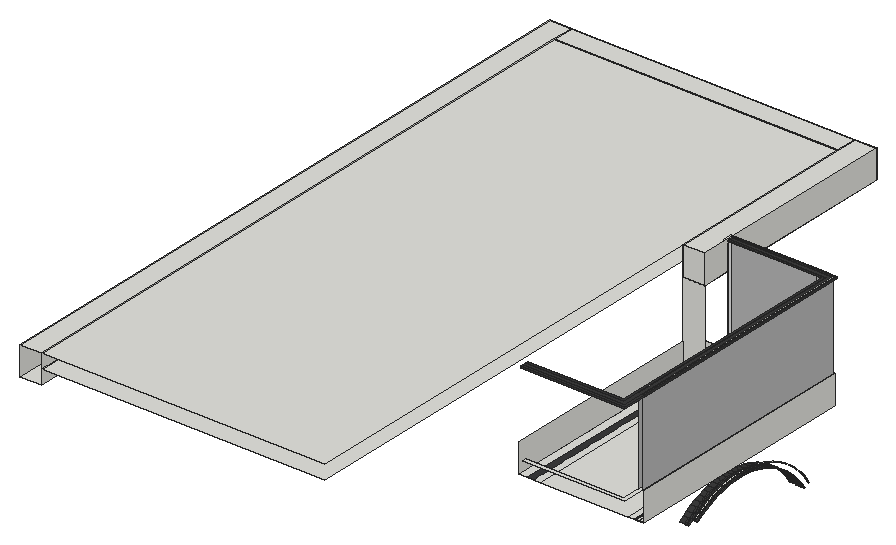
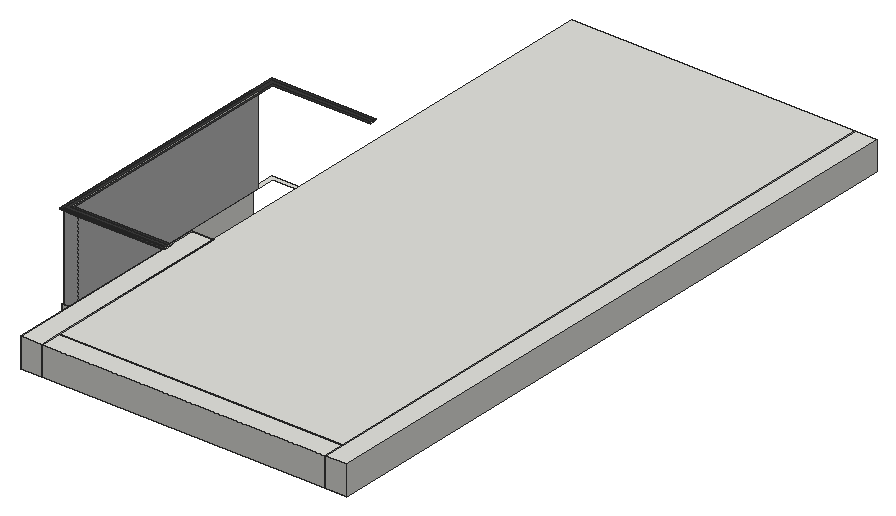
# SketchUp Ruby script. Lengths in inches.
U = 1.inch
M = Sketchup.active_model
def pt(a) = Geom::Point3d.new(a.map { |v| v * U })
def face(e, loops, mat)
  f = e.add_face(loops[0].map { |a| pt(a) })
  loops[1..].each { |l| e.add_face(l.map { |a| pt(a) }).erase! }
  f.material = f.back_material = mat if mat
  f
end
# faces: each face lists its corners as indices into pts; further lists are holes
def faces(e, pts, list, mat = nil) = list.each { |f| face(e, (f[0].is_a?(Array) ? f : [f]).map { |l| l.map { |i| pts[i] } }, mat) }
# xy, xz, yz: faces in a plane at the given z, y or x. An outline is a flat list of corners, or four numbers for a rectangle; further outlines are holes
def ring(l) = l.size == 4 ? [[l[0], l[1]], [l[2], l[1]], [l[2], l[3]], [l[0], l[3]]] : l.each_slice(2).to_a
def flat(e, list, mat, &to3) = list.each { |f| face(e, (f[0].is_a?(Array) ? f : [f]).map { |l| ring(l).map { |u, v| to3.(u, v) } }, mat) }
def xy(e, z, list, mat = nil) = flat(e, list, mat) { |x, y| [x, y, z] }
def xz(e, y, list, mat = nil) = flat(e, list, mat) { |x, z| [x, y, z] }
def yz(e, x, list, mat = nil) = flat(e, list, mat) { |y, z| [x, y, z] }
def lines(e, pts, list) = list.each { |a, b| e.add_line(pt(pts[a]), pt(pts[b])) }
# prism: a flat outline (further loops are holes) pulled along v
def prism(e, loops, v, mat = nil)
  f = face(e, loops, mat); d = Geom::Vector3d.new(v.map { |x| x * U })
  f.pushpull(f.normal.samedirection?(d) ? d.length : -d.length)
end
def box(e, o, s, mat = nil) = prism(e, [[o, [o[0] + s[0], o[1], o[2]], [o[0] + s[0], o[1] + s[1], o[2]], [o[0], o[1] + s[1], o[2]]]], [0, 0, s[2]], mat)
def at(x, y, z, deg = 0) = Geom::Transformation.translation(pt([x, y, z])) * Geom::Transformation.rotation(ORIGIN, Z_AXIS, deg.degrees)
def axes(o, x, y, z) = Geom::Transformation.new([*x, 0, *y, 0, *z, 0, *pt(o).to_a, 1])
def part(name) = M.definitions.add(name)
# library, detail: a bought-in or finely detailed component or shape, given as its bounding box
def library(name, o, s) = part(name).tap { |d| box(d.entities, o, s) }
def detail(e, o, s) = box(e.add_group.entities, o, s)
def put(e, d, t, mat = nil) = e.add_instance(d, t).tap { |i| i.material = mat if mat }
def group(e, t, mat = nil) = e.add_group.tap { |g| g.transformation = t; g.material = mat if mat }.entities
root = M.entities
M.materials.add("[Color M07]").color = [58, 58, 58]
M.materials.add("[Mirror 01]").color = [185, 185, 185]
M.materials.add("[Mirror 02]").color = [229, 229, 229]
xy(root,336.73,[[150.22,149.02,151.47,169.15],[150.22,172.14,151.47,188.97],[150.22,191.96,151.47,209.51]],"[Color M07]")
xy(root,337.6875,[[145.27,124.96,145.27,215.22,190.96,215.22,190.96,124.96,154.46,124.96,154.46,210.47,145.46,210.47,145.46,124.96],[145.46,124.96,148.9,210.47],[151.47,124.96,154.46,210.47],[190.96,124.96,193.21,224.6],[193.21,124.96,193.59,224.6],
  [193.59,124.96,193.96,224.6],[193.96,124.96,194.34,224.6],[194.34,124.96,194.71,224.6],[194.71,124.96,195.09,224.6],[195.09,124.96,195.46,224.6],
  [195.46,124.96,195.84,224.6],[195.84,124.96,196.21,224.6],[196.21,124.96,196.59,224.6],[196.59,124.96,197.34,224.6]])
xy(root,337.6875,[[148.9,124.96,151.47,210.47]],"[Color M07]")
xy(root,349.6875,[[154.46,115.71,154.46,117.49,195.18,117.49,195.18,222.44,154.46,222.44,154.46,224.22,196.96,224.22,196.96,115.71],[196.96,124.96,197.34,224.6],[154.46,224.22,190.96,224.6],[190.96,224.22,196.96,224.6]])
xy(root,373.6875,[[18.46,24,27.46,299.8125],[145.46,210.47,154.46,299.8125],[27.46,290.8125,145.46,299.8125]])
xy(root,379.6875,[[27.46,24,145.46,290.8125]])
xy(root,385.0625,[[154.46,115.71,154.46,117.49,195.18,117.49,195.18,222.44,154.46,222.44,154.46,224.22,196.96,224.22,196.96,115.71]])
xy(root,385.0625,[[154.46,114.76,154.46,115.71,196.96,115.71,196.96,224.22,154.46,224.22,154.46,225.17,197.91,225.17,197.91,114.76]],"[Color M07]")
xy(root,385.6875,[[18.46,24,27.46,299.8125],[27.46,24,145.46,290.8125],[145.46,210.47,154.46,210.47,154.46,221.49,153.51,221.49,153.51,225.17,154.46,225.17,154.46,299.8125,145.46,299.8125],[153.51,221.49,154.46,225.17],[27.46,290.8125,145.46,299.8125]])
xy(root,385.6875,[[154.46,114.76,197.91,114.76,197.91,225.17,154.46,225.17,154.46,224.22,196.96,224.22,196.96,115.71,154.46,115.71],[154.46,115.71,196.96,115.71,196.96,224.22,154.46,224.22,154.46,222.44,195.18,222.44,195.18,117.49,154.46,117.49],[154.46,117.49,195.18,117.49,195.18,222.44,154.46,222.44,154.46,221.49,194.23,221.49,194.23,118.4375,154.46,118.4375]],"[Color M07]")
xz(root,210.47,[[145.46,337.6875,154.46,373.6875],[145.46,373.6875,154.46,385.6875]])
xz(root,215.22,[[145.27,337.6875,154.46,349.6875]])
xz(root,222.44,[[190.96,385.0625,195.18,385.6875]])
xz(root,222.44,[[154.46,385.0625,156.24,385.6875],[156.24,385.0625,190.96,385.6875]],"[Color M07]")
xz(root,222.44,[[156.24,349.6875,190.96,385.0625],[190.96,349.6875,195.18,385.0625]],"[Mirror 01]")
xz(root,222.44,[[154.46,349.6875,156.24,385.0625]],"[Mirror 02]")
xz(root,224.22,[[154.46,385.0625,190.96,385.6875],[190.96,385.0625,196.96,385.6875]])
xz(root,224.22,[[154.46,349.6875,190.96,385.0625],[190.96,349.6875,196.96,385.0625]],"[Mirror 01]")
xz(root,224.6,[[190.96,337.6875,197.34,349.6875]])
xz(root,225.17,[[154.46,385.0625,190.96,385.6875],[190.96,385.0625,197.91,385.6875]],"[Color M07]")
xz(root,290.8125,[[27.46,373.6875,145.46,379.6875],[27.46,379.6875,145.46,385.6875]])
xz(root,299.8125,[[18.46,373.6875,27.46,385.6875],[27.46,373.6875,145.46,385.6875],[145.46,373.6875,154.46,385.6875]])
yz(root,18.46,[[24,373.6875,299.8125,385.6875]])
yz(root,27.46,[[24,373.6875,290.8125,379.6875],[290.8125,373.6875,299.8125,385.6875],[24,379.6875,290.8125,385.6875]])
yz(root,145.27,[[124.96,337.6875,215.22,349.6875]])
yz(root,145.46,[[210.47,373.6875,290.8125,379.6875],[290.8125,373.6875,299.8125,385.6875],[210.47,379.6875,290.8125,385.6875]])
yz(root,154.46,[[222.44,349.6875,224.22,373.6875],[210.47,373.6875,222.44,385.6875],[222.44,373.6875,224.22,385.0625],[224.22,373.6875,299.8125,373.6875,299.8125,385.6875,225.17,385.6875,225.17,385.0625,224.22,385.0625],[222.44,385.0625,224.22,385.6875],
  [224.22,385.0625,225.17,385.6875]])
yz(root,195.18,[[124.96,385.0625,222.44,385.6875]])
yz(root,195.18,[[124.96,349.6875,222.44,385.0625]],"[Mirror 01]")
yz(root,196.96,[[124.96,385.0625,224.22,385.6875]])
yz(root,196.96,[[124.96,349.6875,224.22,385.0625]],"[Mirror 01]")
yz(root,197.34,[[124.96,337.6875,224.6,349.6875]])
yz(root,197.91,[[124.96,385.0625,225.17,385.6875]],"[Color M07]")
p = [[190.96,209.22,313.61],[193.21,209.22,313.61],[193.21,207.91,315.55],[190.96,207.91,315.55],[193.59,207.91,315.55],[193.59,209.22,313.61],
  [193.96,207.91,315.55],[193.96,209.22,313.61],[194.34,207.91,315.55],[194.34,209.22,313.61],[194.71,207.91,315.55],[194.71,209.22,313.61],
  [195.09,207.91,315.55],[195.09,209.22,313.61],[195.46,207.91,315.55],[195.46,209.22,313.61],[195.84,207.91,315.55],[195.84,209.22,313.61],
  [196.21,207.91,315.55],[196.21,209.22,313.61],[196.59,207.91,315.55],[196.59,209.22,313.61],[196.96,207.91,315.55],[196.96,209.22,313.61],
  [196.96,209.77,316.88],[196.96,211.15,314.82],[197.34,211.15,314.82],[197.34,209.77,316.88],[193.21,206.49,317.42],[190.96,206.49,317.42],
  [193.59,206.49,317.42],[193.96,206.49,317.42],[194.34,206.49,317.42],[194.71,206.49,317.42],[195.09,206.49,317.42],[195.46,206.49,317.42],
  [195.84,206.49,317.42],[196.21,206.49,317.42],[196.59,206.49,317.42],[196.96,206.49,317.42],[196.96,208.26,318.85],[197.34,208.26,318.85],
  [193.21,204.96,319.19],[190.96,204.96,319.19],[193.59,204.96,319.19],[193.96,204.96,319.19],[194.34,204.96,319.19],[194.71,204.96,319.19],
  [195.09,204.96,319.19],[195.46,204.96,319.19],[195.84,204.96,319.19],[196.21,204.96,319.19],[196.59,204.96,319.19],[196.96,204.96,319.19],
  [196.96,206.65,320.73],[197.34,206.65,320.73],[193.21,203.33,320.88],[190.96,203.33,320.88],[193.59,203.33,320.88],[193.96,203.33,320.88],
  [194.34,203.33,320.88],[194.71,203.33,320.88],[195.09,203.33,320.88],[195.46,203.33,320.88],[195.84,203.33,320.88],[196.21,203.33,320.88],
  [196.59,203.33,320.88],[196.96,203.33,320.88],[196.96,204.92,322.51],[197.34,204.92,322.51],[193.21,201.6,322.46],[190.96,201.6,322.46],
  [193.59,201.6,322.46],[193.96,201.6,322.46],[194.34,201.6,322.46],[194.71,201.6,322.46],[195.09,201.6,322.46],[195.46,201.6,322.46],
  [195.84,201.6,322.46],[196.21,201.6,322.46],[196.59,201.6,322.46],[196.96,201.6,322.46],[193.21,199.79,323.9375],[190.96,199.79,323.9375],
  [193.59,199.79,323.9375],[193.96,199.79,323.9375],[194.34,199.79,323.9375],[194.71,199.79,323.9375],[195.09,199.79,323.9375],[195.46,199.79,323.9375],
  [195.84,199.79,323.9375],[196.21,199.79,323.9375],[196.59,199.79,323.9375],[196.96,199.79,323.9375],[196.96,203.1,324.1875],[197.34,203.1,324.1875],
  [190.96,153.71,325.31],[193.21,153.71,325.31],[193.21,151.81,323.9375],[190.96,151.81,323.9375],[193.59,151.81,323.9375],[193.59,153.71,325.31],
  [193.96,151.81,323.9375],[193.96,153.71,325.31],[194.34,151.81,323.9375],[194.34,153.71,325.31],[194.71,151.81,323.9375],[194.71,153.71,325.31],
  [193.21,197.88,325.31],[190.96,197.88,325.31],[193.59,197.88,325.31],[193.96,197.88,325.31],[194.34,197.88,325.31],[194.71,197.88,325.31],
  [195.09,197.88,325.31],[195.46,197.88,325.31],[195.84,197.88,325.31],[196.21,197.88,325.31],[196.59,197.88,325.31],[196.96,197.88,325.31],
  [196.96,201.17,325.75],[197.34,201.17,325.75],[190.96,155.69,326.56],[193.21,155.69,326.56],[193.59,155.69,326.56],[193.96,155.69,326.56],
  [194.34,155.69,326.56],[194.71,155.69,326.56],[195.09,153.71,325.31],[195.09,155.69,326.56],[195.46,153.71,325.31],[195.46,155.69,326.56],
  [195.84,153.71,325.31],[195.84,155.69,326.56],[196.21,153.71,325.31],[196.21,155.69,326.56],[196.59,153.71,325.31],[196.59,155.69,326.56],
  [196.96,153.71,325.31],[196.96,155.69,326.56],[193.21,195.9,326.56],[190.96,195.9,326.56],[193.59,195.9,326.56],[193.96,195.9,326.56],
  [194.34,195.9,326.56],[194.71,195.9,326.56],[195.09,195.9,326.56],[195.46,195.9,326.56],[195.84,195.9,326.56],[196.21,195.9,326.56],
  [196.59,195.9,326.56],[196.96,195.9,326.56],[196.96,199.16,327.2],[197.34,199.16,327.2],[190.96,157.74,327.69],[193.21,157.74,327.69],
  [193.59,157.74,327.69],[193.96,157.74,327.69],[194.34,157.74,327.69],[194.71,157.74,327.69],[195.09,157.74,327.69],[195.46,157.74,327.69],
  [195.84,157.74,327.69],[196.21,157.74,327.69],[196.59,157.74,327.69],[196.96,157.74,327.69],[193.21,193.85,327.69],[190.96,193.85,327.69],
  [193.59,193.85,327.69],[193.96,193.85,327.69],[194.34,193.85,327.69],[194.71,193.85,327.69],[195.09,193.85,327.69],[195.46,193.85,327.69],
  [195.84,193.85,327.69],[196.21,193.85,327.69],[196.59,193.85,327.69],[196.96,193.85,327.69],[196.96,152.43,327.2],[196.96,154.53,328.53],
  [197.34,154.53,328.53],[197.34,152.43,327.2],[196.96,197.06,328.53],[197.34,197.06,328.53],[190.96,159.86,328.7],[193.21,159.86,328.7],
  [193.59,159.86,328.7],[193.96,159.86,328.7],[194.34,159.86,328.7],[194.71,159.86,328.7],[195.09,159.86,328.7],[195.46,159.86,328.7],
  [195.84,159.86,328.7],[196.21,159.86,328.7],[196.59,159.86,328.7],[196.96,159.86,328.7],[193.21,191.74,328.7],[190.96,191.74,328.7],
  [193.59,191.74,328.7],[193.96,191.74,328.7],[194.34,191.74,328.7],[194.71,191.74,328.7],[195.09,191.74,328.7],[195.46,191.74,328.7],
  [195.84,191.74,328.7],[196.21,191.74,328.7],[196.59,191.74,328.7],[196.96,191.74,328.7],[196.96,156.7,329.72],[197.34,156.7,329.72],
  [196.96,194.89,329.72],[197.34,194.89,329.72],[190.96,162.03,329.58],[193.21,162.03,329.58],[193.59,162.03,329.58],[193.96,162.03,329.58],
  [194.34,162.03,329.58],[194.71,162.03,329.58],[195.09,162.03,329.58],[195.46,162.03,329.58],[195.84,162.03,329.58],[196.21,162.03,329.58],
  [196.59,162.03,329.58],[196.96,162.03,329.58],[193.21,189.5625,329.58],[190.96,189.5625,329.58],[193.59,189.5625,329.58],[193.96,189.5625,329.58],
  [194.34,189.5625,329.58],[194.71,189.5625,329.58],[195.09,189.5625,329.58],[195.46,189.5625,329.58],[195.84,189.5625,329.58],[196.21,189.5625,329.58],
  [196.59,189.5625,329.58],[196.96,189.5625,329.58],[190.96,164.25,330.34],[193.21,164.25,330.34],[193.59,164.25,330.34],[193.96,164.25,330.34],
  [194.34,164.25,330.34],[194.71,164.25,330.34],[195.09,164.25,330.34],[195.46,164.25,330.34],[195.84,164.25,330.34],[196.21,164.25,330.34],
  [196.59,164.25,330.34],[196.96,164.25,330.34],[193.21,187.34,330.34],[190.96,187.34,330.34],[193.59,187.34,330.34],[193.96,187.34,330.34],
  [194.34,187.34,330.34],[194.71,187.34,330.34],[195.09,187.34,330.34],[195.46,187.34,330.34],[195.84,187.34,330.34],[196.21,187.34,330.34],
  [196.59,187.34,330.34],[196.96,187.34,330.34],[196.96,158.94,330.79],[197.34,158.94,330.79],[196.96,192.66,330.79],[197.34,192.66,330.79],
  [190.96,166.51,330.95],[193.21,166.51,330.95],[193.59,166.51,330.95],[193.96,166.51,330.95],[194.34,166.51,330.95],[194.71,166.51,330.95],
  [195.09,166.51,330.95],[195.46,166.51,330.95],[195.84,166.51,330.95],[196.21,166.51,330.95],[196.59,166.51,330.95],[196.96,166.51,330.95],
  [193.21,185.08,330.95],[190.96,185.08,330.95],[193.59,185.08,330.95],[193.96,185.08,330.95],[194.34,185.08,330.95],[194.71,185.08,330.95],
  [195.09,185.08,330.95],[195.46,185.08,330.95],[195.84,185.08,330.95],[196.21,185.08,330.95],[196.59,185.08,330.95],[196.96,185.08,330.95],
  [196.96,161.23,331.72],[197.34,161.23,331.72],[196.96,190.36,331.72],[197.34,190.36,331.72],[190.96,168.8,331.4375],[193.21,168.8,331.4375],
  [193.59,168.8,331.4375],[193.96,168.8,331.4375],[194.34,168.8,331.4375],[194.71,168.8,331.4375],[195.09,168.8,331.4375],[195.46,168.8,331.4375],
  [195.84,168.8,331.4375],[196.21,168.8,331.4375],[196.59,168.8,331.4375],[196.96,168.8,331.4375],[193.21,182.79,331.4375],[190.96,182.79,331.4375],
  [193.59,182.79,331.4375],[193.96,182.79,331.4375],[194.34,182.79,331.4375],[194.71,182.79,331.4375],[195.09,182.79,331.4375],[195.46,182.79,331.4375],
  [195.84,182.79,331.4375],[196.21,182.79,331.4375],[196.59,182.79,331.4375],[196.96,182.79,331.4375],[190.96,171.12,331.78],[193.21,171.12,331.78],
  [193.59,171.12,331.78],[193.96,171.12,331.78],[194.34,171.12,331.78],[194.71,171.12,331.78],[195.09,171.12,331.78],[195.46,171.12,331.78],
  [195.84,171.12,331.78],[196.21,171.12,331.78],[196.59,171.12,331.78],[196.96,171.12,331.78],[193.21,180.47,331.78],[190.96,180.47,331.78],
  [193.59,180.47,331.78],[193.96,180.47,331.78],[194.34,180.47,331.78],[194.71,180.47,331.78],[195.09,180.47,331.78],[195.46,180.47,331.78],
  [195.84,180.47,331.78],[196.21,180.47,331.78],[196.59,180.47,331.78],[196.96,180.47,331.78],[196.96,163.58,332.52],[197.34,163.58,332.52],
  [196.96,188.01,332.52],[197.34,188.01,332.52],[190.96,173.45,331.99],[193.21,173.45,331.99],[193.59,173.45,331.99],[193.96,173.45,331.99],
  [194.34,173.45,331.99],[194.71,173.45,331.99],[195.09,173.45,331.99],[195.46,173.45,331.99],[195.84,173.45,331.99],[196.21,173.45,331.99],
  [196.59,173.45,331.99],[196.96,173.45,331.99],[193.21,178.14,331.99],[190.96,178.14,331.99],[193.59,178.14,331.99],[193.96,178.14,331.99],
  [194.34,178.14,331.99],[194.71,178.14,331.99],[195.09,178.14,331.99],[195.46,178.14,331.99],[195.84,178.14,331.99],[196.21,178.14,331.99],
  [196.59,178.14,331.99],[196.96,178.14,331.99],[190.96,175.8,332.0625],[193.21,175.8,332.0625],[193.59,175.8,332.0625],[193.96,175.8,332.0625],
  [194.34,175.8,332.0625],[194.71,175.8,332.0625],[195.09,175.8,332.0625],[195.46,175.8,332.0625],[195.84,175.8,332.0625],[196.21,175.8,332.0625],
  [196.59,175.8,332.0625],[196.96,175.8,332.0625],[196.96,165.97,333.17],[197.34,165.97,333.17],[196.96,185.62,333.17],[197.34,185.62,333.17],
  [196.96,168.4,333.6875],[197.34,168.4,333.6875],[196.96,183.2,333.6875],[197.34,183.2,333.6875],[196.96,170.85,334.05],[197.34,170.85,334.05],
  [196.96,180.74,334.05],[197.34,180.74,334.05],[196.96,173.32,334.27],[197.34,173.32,334.27],[196.96,178.27,334.27],[197.34,178.27,334.27],
  [196.96,175.8,334.35],[197.34,175.8,334.35],[190.96,215.22,337.6875],[190.96,215.22,349.6875]]
faces(root,p,[[0,1,2,3],[4,2,1,5],[6,4,5,7],[8,6,7,9],[10,8,9,11],[12,10,11,13],[14,12,13,15],[16,14,15,17],
  [18,16,17,19],[20,18,19,21],[22,20,21,23],[3,2,28,29],[30,28,2,4],[31,30,4,6],[32,31,6,8],[33,32,8,10],
  [34,33,10,12],[35,34,12,14],[36,35,14,16],[37,36,16,18],[38,37,18,20],[39,38,20,22],[29,28,42,43],[44,42,28,30],
  [45,44,30,31],[46,45,31,32],[47,46,32,33],[48,47,33,34],[49,48,34,35],[50,49,35,36],[51,50,36,37],[52,51,37,38],
  [53,52,38,39],[43,42,56,57],[58,56,42,44],[59,58,44,45],[60,59,45,46],[61,60,46,47],[62,61,47,48],[63,62,48,49],
  [64,63,49,50],[65,64,50,51],[66,65,51,52],[67,66,52,53],[57,56,70,71],[72,70,56,58],[73,72,58,59],[74,73,59,60],
  [75,74,60,61],[76,75,61,62],[77,76,62,63],[78,77,63,64],[79,78,64,65],[80,79,65,66],[81,80,66,67],[71,70,82,83],
  [84,82,70,72],[85,84,72,73],[86,85,73,74],[87,86,74,75],[88,87,75,76],[89,88,76,77],[90,89,77,78],[91,90,78,79],
  [92,91,79,80],[93,92,80,81],[96,97,98,99],[100,98,97,101],[102,100,101,103],[104,102,103,105],[106,104,105,107],[83,82,108,109],
  [110,108,82,84],[111,110,84,85],[112,111,85,86],[113,112,86,87],[114,113,87,88],[115,114,88,89],[116,115,89,90],[117,116,90,91],
  [118,117,91,92],[119,118,92,93],[122,123,97,96],[101,97,123,124],[103,101,124,125],[105,103,125,126],[107,105,126,127],[128,107,127,129],
  [130,128,129,131],[132,130,131,133],[134,132,133,135],[136,134,135,137],[138,136,137,139],[109,108,140,141],[142,140,108,110],[143,142,110,111],
  [144,143,111,112],[145,144,112,113],[146,145,113,114],[147,146,114,115],[148,147,115,116],[149,148,116,117],[150,149,117,118],[151,150,118,119],
  [154,155,123,122],[124,123,155,156],[125,124,156,157],[126,125,157,158],[127,126,158,159],[129,127,159,160],[131,129,160,161],[133,131,161,162],
  [135,133,162,163],[137,135,163,164],[139,137,164,165],[141,140,166,167],[168,166,140,142],[169,168,142,143],[170,169,143,144],[171,170,144,145],
  [172,171,145,146],[173,172,146,147],[174,173,147,148],[175,174,148,149],[176,175,149,150],[177,176,150,151],[184,185,155,154],[156,155,185,186],
  [157,156,186,187],[158,157,187,188],[159,158,188,189],[160,159,189,190],[161,160,190,191],[162,161,191,192],[163,162,192,193],[164,163,193,194],
  [165,164,194,195],[167,166,196,197],[198,196,166,168],[199,198,168,169],[200,199,169,170],[201,200,170,171],[202,201,171,172],[203,202,172,173],
  [204,203,173,174],[205,204,174,175],[206,205,175,176],[207,206,176,177],[212,213,185,184],[186,185,213,214],[187,186,214,215],[188,187,215,216],
  [189,188,216,217],[190,189,217,218],[191,190,218,219],[192,191,219,220],[193,192,220,221],[194,193,221,222],[195,194,222,223],[197,196,224,225],
  [226,224,196,198],[227,226,198,199],[228,227,199,200],[229,228,200,201],[230,229,201,202],[231,230,202,203],[232,231,203,204],[233,232,204,205],
  [234,233,205,206],[235,234,206,207],[236,237,213,212],[214,213,237,238],[215,214,238,239],[216,215,239,240],[217,216,240,241],[218,217,241,242],
  [219,218,242,243],[220,219,243,244],[221,220,244,245],[222,221,245,246],[223,222,246,247],[225,224,248,249],[250,248,224,226],[251,250,226,227],
  [252,251,227,228],[253,252,228,229],[254,253,229,230],[255,254,230,231],[256,255,231,232],[257,256,232,233],[258,257,233,234],[259,258,234,235],
  [264,265,237,236],[238,237,265,266],[239,238,266,267],[240,239,267,268],[241,240,268,269],[242,241,269,270],[243,242,270,271],[244,243,271,272],
  [245,244,272,273],[246,245,273,274],[247,246,274,275],[249,248,276,277],[278,276,248,250],[279,278,250,251],[280,279,251,252],[281,280,252,253],
  [282,281,253,254],[283,282,254,255],[284,283,255,256],[285,284,256,257],[286,285,257,258],[287,286,258,259],[292,293,265,264],[266,265,293,294],
  [267,266,294,295],[268,267,295,296],[269,268,296,297],[270,269,297,298],[271,270,298,299],[272,271,299,300],[273,272,300,301],[274,273,301,302],
  [275,274,302,303],[277,276,304,305],[306,304,276,278],[307,306,278,279],[308,307,279,280],[309,308,280,281],[310,309,281,282],[311,310,282,283],
  [312,311,283,284],[313,312,284,285],[314,313,285,286],[315,314,286,287],[316,317,293,292],[294,293,317,318],[295,294,318,319],[296,295,319,320],
  [297,296,320,321],[298,297,321,322],[299,298,322,323],[300,299,323,324],[301,300,324,325],[302,301,325,326],[303,302,326,327],[305,304,328,329],
  [330,328,304,306],[331,330,306,307],[332,331,307,308],[333,332,308,309],[334,333,309,310],[335,334,310,311],[336,335,311,312],[337,336,312,313],
  [338,337,313,314],[339,338,314,315],[344,345,317,316],[318,317,345,346],[319,318,346,347],[320,319,347,348],[321,320,348,349],[322,321,349,350],
  [323,322,350,351],[324,323,351,352],[325,324,352,353],[326,325,353,354],[327,326,354,355],[329,328,356,357],[358,356,328,330],[359,358,330,331],
  [360,359,331,332],[361,360,332,333],[362,361,333,334],[363,362,334,335],[364,363,335,336],[365,364,336,337],[366,365,337,338],[367,366,338,339],
  [368,369,345,344],[346,345,369,370],[347,346,370,371],[348,347,371,372],[349,348,372,373],[350,349,373,374],[351,350,374,375],[352,351,375,376],
  [353,352,376,377],[354,353,377,378],[355,354,378,379],[357,356,369,368],[370,369,356,358],[371,370,358,359],[372,371,359,360],[373,372,360,361],
  [374,373,361,362],[375,374,362,363],[376,375,363,364],[377,376,364,365],[378,377,365,366],[379,378,366,367]],"[Color M07]")
faces(root,p,[[24,25,26,27],[40,24,27,41],[54,40,41,55],[68,54,55,69],[94,68,69,95],[120,94,95,121],[152,120,121,153],[178,179,180,181],
  [182,152,153,183],[179,208,209,180],[210,182,183,211],[208,260,261,209],[262,210,211,263],[260,288,289,261],[290,262,263,291],[288,340,341,289],
  [342,290,291,343],[340,380,381,341],[382,342,343,383],[380,384,385,381],[386,382,383,387],[384,388,389,385],[390,386,387,391],[388,392,393,389],
  [394,390,391,395],[392,396,397,393],[396,394,395,397]])
lines(root,p,[[398,399]])
